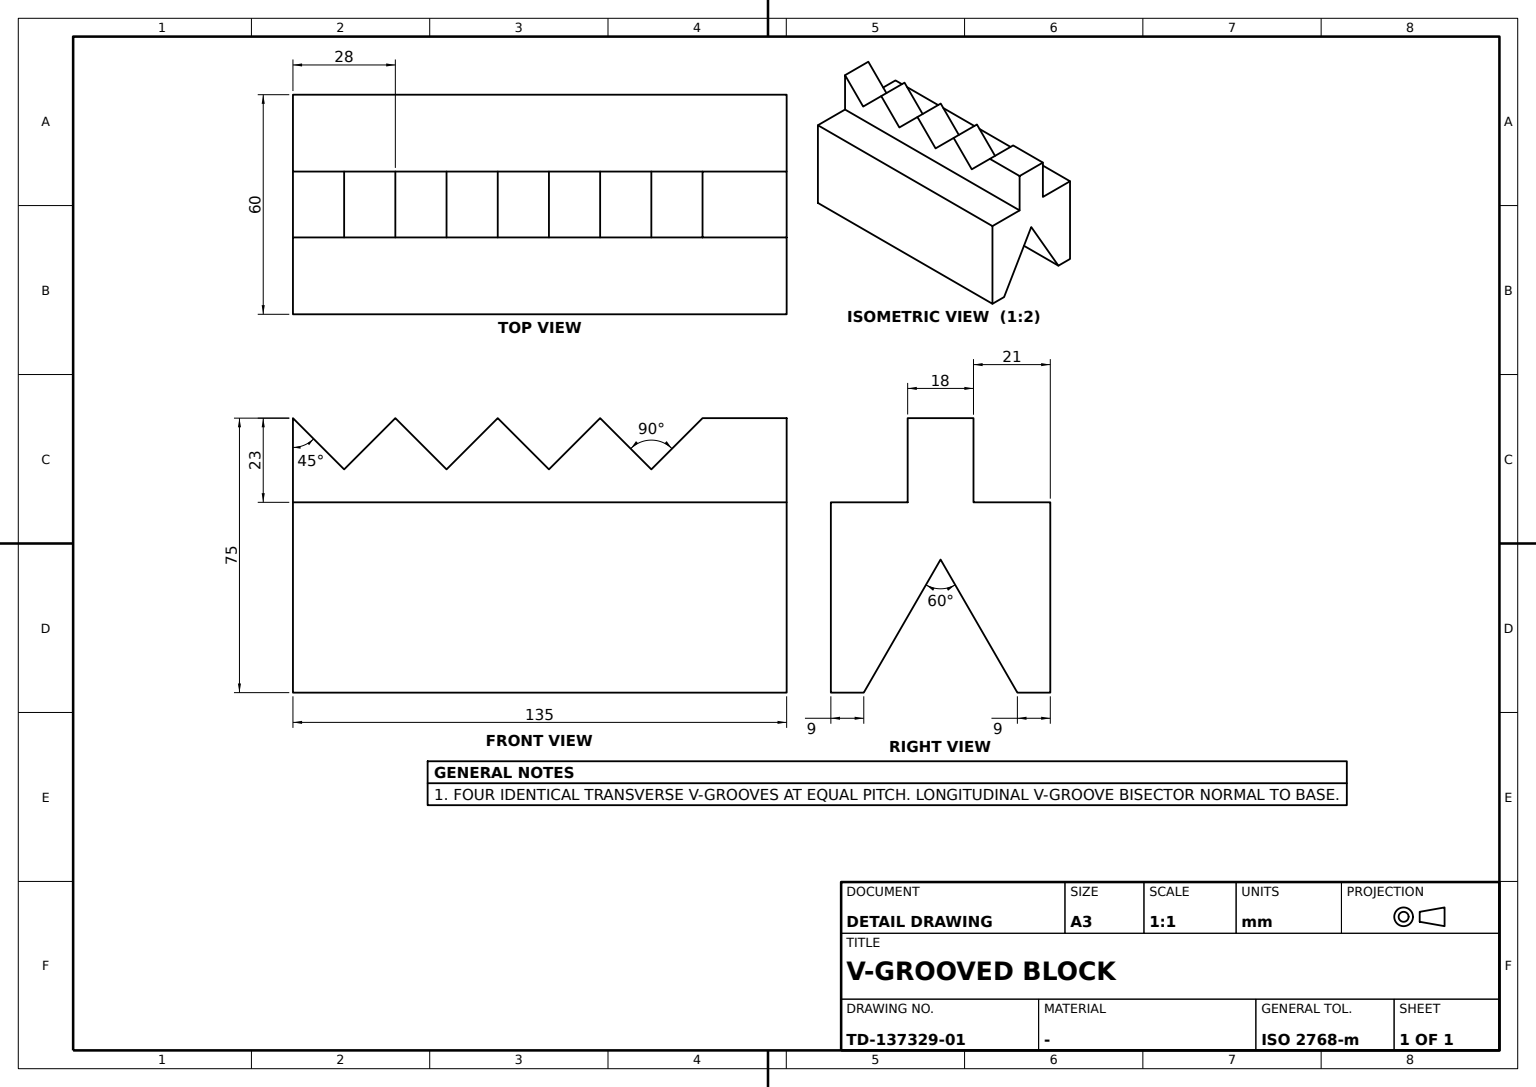
ISO-10303-21;
HEADER;
FILE_DESCRIPTION((''),'2;1');
FILE_NAME('','',(''),(''),'','','');
FILE_SCHEMA(('AUTOMOTIVE_DESIGN'));
ENDSEC;
DATA;
#1=APPLICATION_CONTEXT('');
#2=PRODUCT_CONTEXT('',#1,'mechanical');
#3=PRODUCT('','','',(#2));
#4=PRODUCT_DEFINITION_FORMATION('','',#3);
#5=PRODUCT_DEFINITION_CONTEXT('',#1,'design');
#6=PRODUCT_DEFINITION('','',#4,#5);
#7=PRODUCT_DEFINITION_SHAPE('','',#6);
#8=(LENGTH_UNIT()NAMED_UNIT(*)SI_UNIT(.MILLI.,.METRE.));
#9=(NAMED_UNIT(*)PLANE_ANGLE_UNIT()SI_UNIT($,.RADIAN.));
#10=(NAMED_UNIT(*)SI_UNIT($,.STERADIAN.)SOLID_ANGLE_UNIT());
#11=UNCERTAINTY_MEASURE_WITH_UNIT(LENGTH_MEASURE(0.005),#8,'distance_accuracy_value','');
#12=(GEOMETRIC_REPRESENTATION_CONTEXT(3)GLOBAL_UNCERTAINTY_ASSIGNED_CONTEXT((#11))GLOBAL_UNIT_ASSIGNED_CONTEXT((#8,#9,#10))REPRESENTATION_CONTEXT('',''));
#13=CARTESIAN_POINT('',(9.,-23.,-23.));
#14=VERTEX_POINT('',#13);
#15=CARTESIAN_POINT('',(-9.,-23.,-23.));
#16=VERTEX_POINT('',#15);
#17=CARTESIAN_POINT('',(55000.,-23.,-23.));
#18=DIRECTION('',(-1.,0.,0.));
#19=VECTOR('',#18,1000.);
#20=LINE('',#17,#19);
#21=EDGE_CURVE('',#14,#16,#20,.T.);
#22=ORIENTED_EDGE('',*,*,#21,.F.);
#23=CARTESIAN_POINT('',(9.,-37.,-9.));
#24=VERTEX_POINT('',#23);
#25=CARTESIAN_POINT('',(9.,-11.5,-34.5));
#26=DIRECTION('',(0.,0.707106781,-0.707106781));
#27=VECTOR('',#26,1000.);
#28=LINE('',#25,#27);
#29=EDGE_CURVE('',#24,#14,#28,.T.);
#30=ORIENTED_EDGE('',*,*,#29,.F.);
#31=CARTESIAN_POINT('',(-9.,-37.,-9.));
#32=VERTEX_POINT('',#31);
#33=CARTESIAN_POINT('',(55000.,-37.,-9.));
#34=DIRECTION('',(1.,0.,0.));
#35=VECTOR('',#34,1000.);
#36=LINE('',#33,#35);
#37=EDGE_CURVE('',#32,#24,#36,.T.);
#38=ORIENTED_EDGE('',*,*,#37,.F.);
#39=DIRECTION('',(0.,-0.707106781,0.707106781));
#40=VECTOR('',#39,1000.);
#41=LINE('',#15,#40);
#42=EDGE_CURVE('',#16,#32,#41,.T.);
#43=ORIENTED_EDGE('',*,*,#42,.F.);
#44=EDGE_LOOP('',(#22,#30,#38,#43));
#45=FACE_BOUND('',#44,.T.);
#46=DIRECTION('',(0.,-0.707106781,-0.707106781));
#47=AXIS2_PLACEMENT_3D('',#17,#46,#26);
#48=PLANE('',#47);
#49=ADVANCED_FACE('',(#45),#48,.T.);
#50=CARTESIAN_POINT('',(-30.,-135.,0.));
#51=VERTEX_POINT('',#50);
#52=CARTESIAN_POINT('',(-9.,-135.,0.));
#53=VERTEX_POINT('',#52);
#54=LINE('',#50,#35);
#55=EDGE_CURVE('',#51,#53,#54,.T.);
#56=ORIENTED_EDGE('',*,*,#55,.F.);
#57=CARTESIAN_POINT('',(-30.,0.,0.));
#58=VERTEX_POINT('',#57);
#59=DIRECTION('',(0.,-1.,0.));
#60=VECTOR('',#59,1000.);
#61=LINE('',#57,#60);
#62=EDGE_CURVE('',#58,#51,#61,.T.);
#63=ORIENTED_EDGE('',*,*,#62,.F.);
#64=CARTESIAN_POINT('',(-9.,0.,0.));
#65=VERTEX_POINT('',#64);
#66=LINE('',#57,#35);
#67=EDGE_CURVE('',#58,#65,#66,.T.);
#68=ORIENTED_EDGE('',*,*,#67,.T.);
#69=LINE('',#64,#60);
#70=EDGE_CURVE('',#65,#53,#69,.T.);
#71=ORIENTED_EDGE('',*,*,#70,.T.);
#72=EDGE_LOOP('',(#56,#63,#68,#71));
#73=FACE_BOUND('',#72,.T.);
#74=DIRECTION('',(0.,0.,-1.));
#75=AXIS2_PLACEMENT_3D('',#57,#74,#18);
#76=PLANE('',#75);
#77=ADVANCED_FACE('',(#73),#76,.T.);
#78=CARTESIAN_POINT('',(9.,-79.,-23.));
#79=VERTEX_POINT('',#78);
#80=CARTESIAN_POINT('',(9.,-65.,-9.));
#81=VERTEX_POINT('',#80);
#82=CARTESIAN_POINT('',(9.,-39.5,16.5));
#83=DIRECTION('',(0.,0.707106781,0.707106781));
#84=VECTOR('',#83,1000.);
#85=LINE('',#82,#84);
#86=EDGE_CURVE('',#79,#81,#85,.T.);
#87=ORIENTED_EDGE('',*,*,#86,.F.);
#88=CARTESIAN_POINT('',(-9.,-79.,-23.));
#89=VERTEX_POINT('',#88);
#90=CARTESIAN_POINT('',(55000.,-79.,-23.));
#91=LINE('',#90,#35);
#92=EDGE_CURVE('',#89,#79,#91,.T.);
#93=ORIENTED_EDGE('',*,*,#92,.F.);
#94=CARTESIAN_POINT('',(-9.,-65.,-9.));
#95=VERTEX_POINT('',#94);
#96=CARTESIAN_POINT('',(-9.,-28.,28.));
#97=VECTOR('',#46,1000.);
#98=LINE('',#96,#97);
#99=EDGE_CURVE('',#95,#89,#98,.T.);
#100=ORIENTED_EDGE('',*,*,#99,.F.);
#101=CARTESIAN_POINT('',(55000.,-65.,-9.));
#102=LINE('',#101,#35);
#103=EDGE_CURVE('',#95,#81,#102,.T.);
#104=ORIENTED_EDGE('',*,*,#103,.T.);
#105=EDGE_LOOP('',(#87,#93,#100,#104));
#106=FACE_BOUND('',#105,.T.);
#107=AXIS2_PLACEMENT_3D('',#101,#26,#83);
#108=PLANE('',#107);
#109=ADVANCED_FACE('',(#106),#108,.T.);
#110=CARTESIAN_POINT('',(-9.,-107.,-23.));
#111=VERTEX_POINT('',#110);
#112=CARTESIAN_POINT('',(-9.,-121.,-9.));
#113=VERTEX_POINT('',#112);
#114=CARTESIAN_POINT('',(-9.,-65.,-65.));
#115=LINE('',#114,#40);
#116=EDGE_CURVE('',#111,#113,#115,.T.);
#117=ORIENTED_EDGE('',*,*,#116,.F.);
#118=CARTESIAN_POINT('',(9.,-107.,-23.));
#119=VERTEX_POINT('',#118);
#120=CARTESIAN_POINT('',(55000.,-107.,-23.));
#121=LINE('',#120,#35);
#122=EDGE_CURVE('',#111,#119,#121,.T.);
#123=ORIENTED_EDGE('',*,*,#122,.T.);
#124=CARTESIAN_POINT('',(9.,-121.,-9.));
#125=VERTEX_POINT('',#124);
#126=CARTESIAN_POINT('',(9.,-53.5,-76.5));
#127=LINE('',#126,#27);
#128=EDGE_CURVE('',#125,#119,#127,.T.);
#129=ORIENTED_EDGE('',*,*,#128,.F.);
#130=CARTESIAN_POINT('',(55000.,-121.,-9.));
#131=LINE('',#130,#35);
#132=EDGE_CURVE('',#113,#125,#131,.T.);
#133=ORIENTED_EDGE('',*,*,#132,.F.);
#134=EDGE_LOOP('',(#117,#123,#129,#133));
#135=FACE_BOUND('',#134,.T.);
#136=AXIS2_PLACEMENT_3D('',#120,#46,#26);
#137=PLANE('',#136);
#138=ADVANCED_FACE('',(#135),#137,.T.);
#139=CARTESIAN_POINT('',(-30.,0.,52.));
#140=VERTEX_POINT('',#139);
#141=VECTOR('',#74,1000.);
#142=LINE('',#139,#141);
#143=EDGE_CURVE('',#140,#58,#142,.T.);
#144=ORIENTED_EDGE('',*,*,#143,.T.);
#145=ORIENTED_EDGE('',*,*,#62,.T.);
#146=CARTESIAN_POINT('',(-30.,-135.,52.));
#147=VERTEX_POINT('',#146);
#148=LINE('',#146,#141);
#149=EDGE_CURVE('',#147,#51,#148,.T.);
#150=ORIENTED_EDGE('',*,*,#149,.F.);
#151=LINE('',#139,#60);
#152=EDGE_CURVE('',#140,#147,#151,.T.);
#153=ORIENTED_EDGE('',*,*,#152,.F.);
#154=EDGE_LOOP('',(#144,#145,#150,#153));
#155=FACE_BOUND('',#154,.T.);
#156=DIRECTION('',(0.,0.,1.));
#157=AXIS2_PLACEMENT_3D('',#139,#18,#156);
#158=PLANE('',#157);
#159=ADVANCED_FACE('',(#155),#158,.T.);
#160=CARTESIAN_POINT('',(-9.,-135.,-23.));
#161=VERTEX_POINT('',#160);
#162=LINE('',#52,#141);
#163=EDGE_CURVE('',#53,#161,#162,.T.);
#164=ORIENTED_EDGE('',*,*,#163,.T.);
#165=CARTESIAN_POINT('',(9.,-135.,-23.));
#166=VERTEX_POINT('',#165);
#167=CARTESIAN_POINT('',(0.,-135.,-23.));
#168=LINE('',#167,#35);
#169=EDGE_CURVE('',#161,#166,#168,.T.);
#170=ORIENTED_EDGE('',*,*,#169,.T.);
#171=CARTESIAN_POINT('',(9.,-135.,0.));
#172=VERTEX_POINT('',#171);
#173=VECTOR('',#156,1000.);
#174=LINE('',#165,#173);
#175=EDGE_CURVE('',#166,#172,#174,.T.);
#176=ORIENTED_EDGE('',*,*,#175,.T.);
#177=CARTESIAN_POINT('',(30.,-135.,0.));
#178=VERTEX_POINT('',#177);
#179=LINE('',#171,#35);
#180=EDGE_CURVE('',#172,#178,#179,.T.);
#181=ORIENTED_EDGE('',*,*,#180,.T.);
#182=CARTESIAN_POINT('',(30.,-135.,52.));
#183=VERTEX_POINT('',#182);
#184=LINE('',#177,#173);
#185=EDGE_CURVE('',#178,#183,#184,.T.);
#186=ORIENTED_EDGE('',*,*,#185,.T.);
#187=CARTESIAN_POINT('',(21.,-135.,52.));
#188=VERTEX_POINT('',#187);
#189=LINE('',#182,#19);
#190=EDGE_CURVE('',#183,#188,#189,.T.);
#191=ORIENTED_EDGE('',*,*,#190,.T.);
#192=CARTESIAN_POINT('',(0.,-135.,15.626933));
#193=VERTEX_POINT('',#192);
#194=DIRECTION('',(-0.5,0.,-0.866025404));
#195=VECTOR('',#194,1000.);
#196=LINE('',#187,#195);
#197=EDGE_CURVE('',#188,#193,#196,.T.);
#198=ORIENTED_EDGE('',*,*,#197,.T.);
#199=CARTESIAN_POINT('',(-21.,-135.,52.));
#200=VERTEX_POINT('',#199);
#201=DIRECTION('',(-0.5,0.,0.866025404));
#202=VECTOR('',#201,1000.);
#203=LINE('',#192,#202);
#204=EDGE_CURVE('',#193,#200,#203,.T.);
#205=ORIENTED_EDGE('',*,*,#204,.T.);
#206=LINE('',#199,#19);
#207=EDGE_CURVE('',#200,#147,#206,.T.);
#208=ORIENTED_EDGE('',*,*,#207,.T.);
#209=ORIENTED_EDGE('',*,*,#149,.T.);
#210=ORIENTED_EDGE('',*,*,#55,.T.);
#211=EDGE_LOOP('',(#164,#170,#176,#181,#186,#191,#198,#205,#208,#209,#210));
#212=FACE_BOUND('',#211,.T.);
#213=CARTESIAN_POINT('',(0.,-135.,0.));
#214=AXIS2_PLACEMENT_3D('',#213,#59,#74);
#215=PLANE('',#214);
#216=ADVANCED_FACE('',(#212),#215,.T.);
#217=ORIENTED_EDGE('',*,*,#152,.T.);
#218=ORIENTED_EDGE('',*,*,#207,.F.);
#219=CARTESIAN_POINT('',(-21.,0.,52.));
#220=VERTEX_POINT('',#219);
#221=LINE('',#219,#60);
#222=EDGE_CURVE('',#220,#200,#221,.T.);
#223=ORIENTED_EDGE('',*,*,#222,.F.);
#224=LINE('',#219,#19);
#225=EDGE_CURVE('',#220,#140,#224,.T.);
#226=ORIENTED_EDGE('',*,*,#225,.T.);
#227=EDGE_LOOP('',(#217,#218,#223,#226));
#228=FACE_BOUND('',#227,.T.);
#229=AXIS2_PLACEMENT_3D('',#219,#156,#34);
#230=PLANE('',#229);
#231=ADVANCED_FACE('',(#228),#230,.T.);
#232=CARTESIAN_POINT('',(9.,0.,0.));
#233=VERTEX_POINT('',#232);
#234=CARTESIAN_POINT('',(30.,0.,0.));
#235=VERTEX_POINT('',#234);
#236=LINE('',#232,#35);
#237=EDGE_CURVE('',#233,#235,#236,.T.);
#238=ORIENTED_EDGE('',*,*,#237,.T.);
#239=LINE('',#234,#60);
#240=EDGE_CURVE('',#235,#178,#239,.T.);
#241=ORIENTED_EDGE('',*,*,#240,.T.);
#242=ORIENTED_EDGE('',*,*,#180,.F.);
#243=LINE('',#232,#60);
#244=EDGE_CURVE('',#233,#172,#243,.T.);
#245=ORIENTED_EDGE('',*,*,#244,.F.);
#246=EDGE_LOOP('',(#238,#241,#242,#245));
#247=FACE_BOUND('',#246,.T.);
#248=AXIS2_PLACEMENT_3D('',#232,#74,#18);
#249=PLANE('',#248);
#250=ADVANCED_FACE('',(#247),#249,.T.);
#251=CARTESIAN_POINT('',(9.,-93.,-9.));
#252=VERTEX_POINT('',#251);
#253=CARTESIAN_POINT('',(9.,-39.5,-62.5));
#254=LINE('',#253,#27);
#255=EDGE_CURVE('',#252,#79,#254,.T.);
#256=ORIENTED_EDGE('',*,*,#255,.F.);
#257=CARTESIAN_POINT('',(-9.,-93.,-9.));
#258=VERTEX_POINT('',#257);
#259=CARTESIAN_POINT('',(55000.,-93.,-9.));
#260=LINE('',#259,#35);
#261=EDGE_CURVE('',#258,#252,#260,.T.);
#262=ORIENTED_EDGE('',*,*,#261,.F.);
#263=CARTESIAN_POINT('',(-9.,-51.,-51.));
#264=LINE('',#263,#40);
#265=EDGE_CURVE('',#89,#258,#264,.T.);
#266=ORIENTED_EDGE('',*,*,#265,.F.);
#267=ORIENTED_EDGE('',*,*,#92,.T.);
#268=EDGE_LOOP('',(#256,#262,#266,#267));
#269=FACE_BOUND('',#268,.T.);
#270=AXIS2_PLACEMENT_3D('',#90,#46,#26);
#271=PLANE('',#270);
#272=ADVANCED_FACE('',(#269),#271,.T.);
#273=CARTESIAN_POINT('',(-9.,0.,-23.));
#274=VERTEX_POINT('',#273);
#275=CARTESIAN_POINT('',(9.,0.,-23.));
#276=VERTEX_POINT('',#275);
#277=LINE('',#273,#35);
#278=EDGE_CURVE('',#274,#276,#277,.T.);
#279=ORIENTED_EDGE('',*,*,#278,.T.);
#280=LINE('',#275,#60);
#281=EDGE_CURVE('',#276,#14,#280,.T.);
#282=ORIENTED_EDGE('',*,*,#281,.T.);
#283=ORIENTED_EDGE('',*,*,#21,.T.);
#284=LINE('',#273,#60);
#285=EDGE_CURVE('',#274,#16,#284,.T.);
#286=ORIENTED_EDGE('',*,*,#285,.F.);
#287=EDGE_LOOP('',(#279,#282,#283,#286));
#288=FACE_BOUND('',#287,.T.);
#289=CARTESIAN_POINT('',(0.,0.,-23.));
#290=AXIS2_PLACEMENT_3D('',#289,#74,#18);
#291=PLANE('',#290);
#292=ADVANCED_FACE('',(#288),#291,.T.);
#293=CARTESIAN_POINT('',(-9.,-56.,56.));
#294=LINE('',#293,#97);
#295=EDGE_CURVE('',#113,#161,#294,.T.);
#296=ORIENTED_EDGE('',*,*,#295,.F.);
#297=ORIENTED_EDGE('',*,*,#132,.T.);
#298=CARTESIAN_POINT('',(9.,-67.5,44.5));
#299=LINE('',#298,#84);
#300=EDGE_CURVE('',#166,#125,#299,.T.);
#301=ORIENTED_EDGE('',*,*,#300,.F.);
#302=ORIENTED_EDGE('',*,*,#169,.F.);
#303=EDGE_LOOP('',(#296,#297,#301,#302));
#304=FACE_BOUND('',#303,.T.);
#305=AXIS2_PLACEMENT_3D('',#130,#26,#83);
#306=PLANE('',#305);
#307=ADVANCED_FACE('',(#304),#306,.T.);
#308=CARTESIAN_POINT('',(0.,0.,15.626933));
#309=VERTEX_POINT('',#308);
#310=LINE('',#308,#60);
#311=EDGE_CURVE('',#309,#193,#310,.T.);
#312=ORIENTED_EDGE('',*,*,#311,.T.);
#313=ORIENTED_EDGE('',*,*,#197,.F.);
#314=CARTESIAN_POINT('',(21.,0.,52.));
#315=VERTEX_POINT('',#314);
#316=LINE('',#314,#60);
#317=EDGE_CURVE('',#315,#188,#316,.T.);
#318=ORIENTED_EDGE('',*,*,#317,.F.);
#319=LINE('',#314,#195);
#320=EDGE_CURVE('',#315,#309,#319,.T.);
#321=ORIENTED_EDGE('',*,*,#320,.T.);
#322=EDGE_LOOP('',(#312,#313,#318,#321));
#323=FACE_BOUND('',#322,.T.);
#324=DIRECTION('',(-0.866025404,0.,0.5));
#325=DIRECTION('',(0.5,0.,0.866025404));
#326=AXIS2_PLACEMENT_3D('',#314,#324,#325);
#327=PLANE('',#326);
#328=ADVANCED_FACE('',(#323),#327,.T.);
#329=ORIENTED_EDGE('',*,*,#122,.F.);
#330=CARTESIAN_POINT('',(-9.,-42.,42.));
#331=LINE('',#330,#97);
#332=EDGE_CURVE('',#258,#111,#331,.T.);
#333=ORIENTED_EDGE('',*,*,#332,.F.);
#334=ORIENTED_EDGE('',*,*,#261,.T.);
#335=CARTESIAN_POINT('',(9.,-53.5,30.5));
#336=LINE('',#335,#84);
#337=EDGE_CURVE('',#119,#252,#336,.T.);
#338=ORIENTED_EDGE('',*,*,#337,.F.);
#339=EDGE_LOOP('',(#329,#333,#334,#338));
#340=FACE_BOUND('',#339,.T.);
#341=AXIS2_PLACEMENT_3D('',#259,#26,#83);
#342=PLANE('',#341);
#343=ADVANCED_FACE('',(#340),#342,.T.);
#344=ORIENTED_EDGE('',*,*,#103,.F.);
#345=CARTESIAN_POINT('',(-9.,-51.,-23.));
#346=VERTEX_POINT('',#345);
#347=CARTESIAN_POINT('',(-9.,-37.,-37.));
#348=LINE('',#347,#40);
#349=EDGE_CURVE('',#346,#95,#348,.T.);
#350=ORIENTED_EDGE('',*,*,#349,.F.);
#351=CARTESIAN_POINT('',(9.,-51.,-23.));
#352=VERTEX_POINT('',#351);
#353=CARTESIAN_POINT('',(55000.,-51.,-23.));
#354=LINE('',#353,#35);
#355=EDGE_CURVE('',#346,#352,#354,.T.);
#356=ORIENTED_EDGE('',*,*,#355,.T.);
#357=CARTESIAN_POINT('',(9.,-25.5,-48.5));
#358=LINE('',#357,#27);
#359=EDGE_CURVE('',#81,#352,#358,.T.);
#360=ORIENTED_EDGE('',*,*,#359,.F.);
#361=EDGE_LOOP('',(#344,#350,#356,#360));
#362=FACE_BOUND('',#361,.T.);
#363=AXIS2_PLACEMENT_3D('',#353,#46,#26);
#364=PLANE('',#363);
#365=ADVANCED_FACE('',(#362),#364,.T.);
#366=ORIENTED_EDGE('',*,*,#42,.T.);
#367=CARTESIAN_POINT('',(-9.,-14.,14.));
#368=LINE('',#367,#97);
#369=EDGE_CURVE('',#32,#346,#368,.T.);
#370=ORIENTED_EDGE('',*,*,#369,.T.);
#371=ORIENTED_EDGE('',*,*,#349,.T.);
#372=ORIENTED_EDGE('',*,*,#99,.T.);
#373=ORIENTED_EDGE('',*,*,#265,.T.);
#374=ORIENTED_EDGE('',*,*,#332,.T.);
#375=ORIENTED_EDGE('',*,*,#116,.T.);
#376=ORIENTED_EDGE('',*,*,#295,.T.);
#377=ORIENTED_EDGE('',*,*,#163,.F.);
#378=ORIENTED_EDGE('',*,*,#70,.F.);
#379=LINE('',#64,#141);
#380=EDGE_CURVE('',#65,#274,#379,.T.);
#381=ORIENTED_EDGE('',*,*,#380,.T.);
#382=ORIENTED_EDGE('',*,*,#285,.T.);
#383=EDGE_LOOP('',(#366,#370,#371,#372,#373,#374,#375,#376,#377,#378,#381,#382));
#384=FACE_BOUND('',#383,.T.);
#385=AXIS2_PLACEMENT_3D('',#64,#18,#156);
#386=PLANE('',#385);
#387=ADVANCED_FACE('',(#384),#386,.T.);
#388=ORIENTED_EDGE('',*,*,#240,.F.);
#389=CARTESIAN_POINT('',(30.,0.,52.));
#390=VERTEX_POINT('',#389);
#391=LINE('',#234,#173);
#392=EDGE_CURVE('',#235,#390,#391,.T.);
#393=ORIENTED_EDGE('',*,*,#392,.T.);
#394=LINE('',#389,#60);
#395=EDGE_CURVE('',#390,#183,#394,.T.);
#396=ORIENTED_EDGE('',*,*,#395,.T.);
#397=ORIENTED_EDGE('',*,*,#185,.F.);
#398=EDGE_LOOP('',(#388,#393,#396,#397));
#399=FACE_BOUND('',#398,.T.);
#400=AXIS2_PLACEMENT_3D('',#234,#34,#74);
#401=PLANE('',#400);
#402=ADVANCED_FACE('',(#399),#401,.T.);
#403=ORIENTED_EDGE('',*,*,#37,.T.);
#404=CARTESIAN_POINT('',(9.,-25.5,2.5));
#405=LINE('',#404,#84);
#406=EDGE_CURVE('',#352,#24,#405,.T.);
#407=ORIENTED_EDGE('',*,*,#406,.F.);
#408=ORIENTED_EDGE('',*,*,#355,.F.);
#409=ORIENTED_EDGE('',*,*,#369,.F.);
#410=EDGE_LOOP('',(#403,#407,#408,#409));
#411=FACE_BOUND('',#410,.T.);
#412=AXIS2_PLACEMENT_3D('',#33,#26,#83);
#413=PLANE('',#412);
#414=ADVANCED_FACE('',(#411),#413,.T.);
#415=ORIENTED_EDGE('',*,*,#222,.T.);
#416=ORIENTED_EDGE('',*,*,#204,.F.);
#417=ORIENTED_EDGE('',*,*,#311,.F.);
#418=LINE('',#308,#202);
#419=EDGE_CURVE('',#309,#220,#418,.T.);
#420=ORIENTED_EDGE('',*,*,#419,.T.);
#421=EDGE_LOOP('',(#415,#416,#417,#420));
#422=FACE_BOUND('',#421,.T.);
#423=DIRECTION('',(0.866025404,0.,0.5));
#424=DIRECTION('',(0.5,0.,-0.866025404));
#425=AXIS2_PLACEMENT_3D('',#308,#423,#424);
#426=PLANE('',#425);
#427=ADVANCED_FACE('',(#422),#426,.T.);
#428=ORIENTED_EDGE('',*,*,#380,.F.);
#429=ORIENTED_EDGE('',*,*,#67,.F.);
#430=ORIENTED_EDGE('',*,*,#143,.F.);
#431=ORIENTED_EDGE('',*,*,#225,.F.);
#432=ORIENTED_EDGE('',*,*,#419,.F.);
#433=ORIENTED_EDGE('',*,*,#320,.F.);
#434=LINE('',#389,#19);
#435=EDGE_CURVE('',#390,#315,#434,.T.);
#436=ORIENTED_EDGE('',*,*,#435,.F.);
#437=ORIENTED_EDGE('',*,*,#392,.F.);
#438=ORIENTED_EDGE('',*,*,#237,.F.);
#439=LINE('',#275,#173);
#440=EDGE_CURVE('',#276,#233,#439,.T.);
#441=ORIENTED_EDGE('',*,*,#440,.F.);
#442=ORIENTED_EDGE('',*,*,#278,.F.);
#443=EDGE_LOOP('',(#428,#429,#430,#431,#432,#433,#436,#437,#438,#441,#442));
#444=FACE_BOUND('',#443,.T.);
#445=CARTESIAN_POINT('',(0.,0.,0.));
#446=AXIS2_PLACEMENT_3D('',#445,#59,#74);
#447=PLANE('',#446);
#448=ADVANCED_FACE('',(#444),#447,.F.);
#449=ORIENTED_EDGE('',*,*,#255,.T.);
#450=ORIENTED_EDGE('',*,*,#86,.T.);
#451=ORIENTED_EDGE('',*,*,#359,.T.);
#452=ORIENTED_EDGE('',*,*,#406,.T.);
#453=ORIENTED_EDGE('',*,*,#29,.T.);
#454=ORIENTED_EDGE('',*,*,#281,.F.);
#455=ORIENTED_EDGE('',*,*,#440,.T.);
#456=ORIENTED_EDGE('',*,*,#244,.T.);
#457=ORIENTED_EDGE('',*,*,#175,.F.);
#458=ORIENTED_EDGE('',*,*,#300,.T.);
#459=ORIENTED_EDGE('',*,*,#128,.T.);
#460=ORIENTED_EDGE('',*,*,#337,.T.);
#461=EDGE_LOOP('',(#449,#450,#451,#452,#453,#454,#455,#456,#457,#458,#459,#460));
#462=FACE_BOUND('',#461,.T.);
#463=AXIS2_PLACEMENT_3D('',#275,#34,#74);
#464=PLANE('',#463);
#465=ADVANCED_FACE('',(#462),#464,.T.);
#466=ORIENTED_EDGE('',*,*,#317,.T.);
#467=ORIENTED_EDGE('',*,*,#190,.F.);
#468=ORIENTED_EDGE('',*,*,#395,.F.);
#469=ORIENTED_EDGE('',*,*,#435,.T.);
#470=EDGE_LOOP('',(#466,#467,#468,#469));
#471=FACE_BOUND('',#470,.T.);
#472=AXIS2_PLACEMENT_3D('',#389,#156,#34);
#473=PLANE('',#472);
#474=ADVANCED_FACE('',(#471),#473,.T.);
#475=CLOSED_SHELL('',(#49,#77,#109,#138,#159,#216,#231,#250,#272,#292,#307,#328,#343,#365,#387,#402,#414,#427,#448,#465,#474));
#476=MANIFOLD_SOLID_BREP('',#475);
#477=ADVANCED_BREP_SHAPE_REPRESENTATION('',(#476),#12);
#478=SHAPE_DEFINITION_REPRESENTATION(#7,#477);
ENDSEC;
END-ISO-10303-21;
